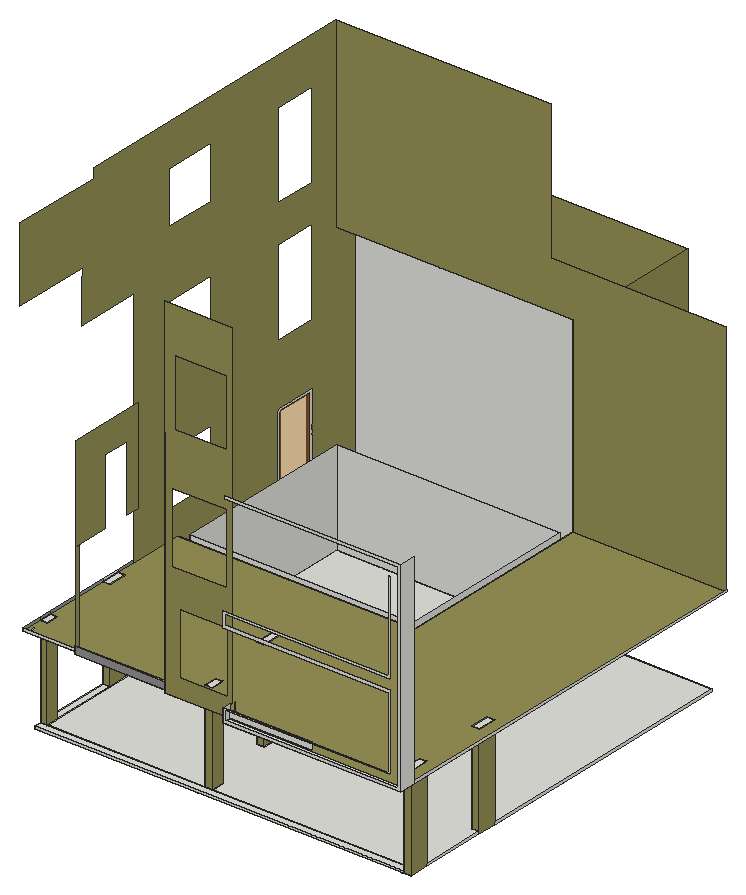
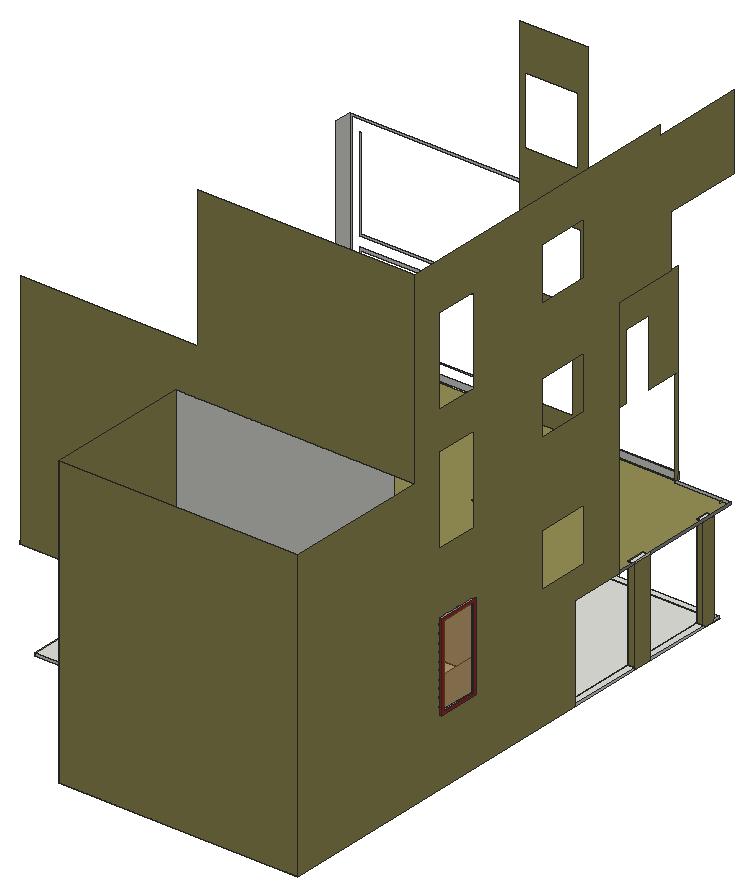
# SketchUp Ruby script. Lengths in inches.
U = 1.inch
M = Sketchup.active_model
def pt(a) = Geom::Point3d.new(a.map { |v| v * U })
def face(e, loops, mat)
  f = e.add_face(loops[0].map { |a| pt(a) })
  loops[1..].each { |l| e.add_face(l.map { |a| pt(a) }).erase! }
  f.material = f.back_material = mat if mat
  f
end
# faces: each face lists its corners as indices into pts; further lists are holes
def faces(e, pts, list, mat = nil) = list.each { |f| face(e, (f[0].is_a?(Array) ? f : [f]).map { |l| l.map { |i| pts[i] } }, mat) }
# xy, xz, yz: faces in a plane at the given z, y or x. An outline is a flat list of corners, or four numbers for a rectangle; further outlines are holes
def ring(l) = l.size == 4 ? [[l[0], l[1]], [l[2], l[1]], [l[2], l[3]], [l[0], l[3]]] : l.each_slice(2).to_a
def flat(e, list, mat, &to3) = list.each { |f| face(e, (f[0].is_a?(Array) ? f : [f]).map { |l| ring(l).map { |u, v| to3.(u, v) } }, mat) }
def xy(e, z, list, mat = nil) = flat(e, list, mat) { |x, y| [x, y, z] }
def xz(e, y, list, mat = nil) = flat(e, list, mat) { |x, z| [x, y, z] }
def yz(e, x, list, mat = nil) = flat(e, list, mat) { |y, z| [x, y, z] }
def lines(e, pts, list) = list.each { |a, b| e.add_line(pt(pts[a]), pt(pts[b])) }
# prism: a flat outline (further loops are holes) pulled along v
def prism(e, loops, v, mat = nil)
  f = face(e, loops, mat); d = Geom::Vector3d.new(v.map { |x| x * U })
  f.pushpull(f.normal.samedirection?(d) ? d.length : -d.length)
end
def box(e, o, s, mat = nil) = prism(e, [[o, [o[0] + s[0], o[1], o[2]], [o[0] + s[0], o[1] + s[1], o[2]], [o[0], o[1] + s[1], o[2]]]], [0, 0, s[2]], mat)
def at(x, y, z, deg = 0) = Geom::Transformation.translation(pt([x, y, z])) * Geom::Transformation.rotation(ORIGIN, Z_AXIS, deg.degrees)
def axes(o, x, y, z) = Geom::Transformation.new([*x, 0, *y, 0, *z, 0, *pt(o).to_a, 1])
def part(name) = M.definitions.add(name)
# library, detail: a bought-in or finely detailed component or shape, given as its bounding box
def library(name, o, s) = part(name).tap { |d| box(d.entities, o, s) }
def detail(e, o, s) = box(e.add_group.entities, o, s)
def put(e, d, t, mat = nil) = e.add_instance(d, t).tap { |i| i.material = mat if mat }
def group(e, t, mat = nil) = e.add_group.tap { |g| g.transformation = t; g.material = mat if mat }.entities
root = M.entities
M.materials.add("[0018_Brown]").color = [165, 42, 42]
M.materials.add("[0057_DarkKhaki]").color = [150, 145, 85]
M.materials.add("[0134_DimGray]").color = [105, 105, 105]
M.materials.add("[Color M05]").color = [145, 145, 145]
M.materials.add("[Translucent Glass Gray]").color = [191, 123, 24]
M.materials["[Translucent Glass Gray]"].alpha = 0.5
xy(root,0,[[12.25,40.75,21.25,40.875],[21.25,40.75,222.625,40.875],[222.625,40.75,482.875,40.875],[11.875,40.875,12.25,65.96],[12.25,40.875,21.25,41.91],
  [21.25,40.875,222.625,49.875],[222.625,40.875,482.875,49.875],[482.875,40.875,491.875,41.91],[12.25,41.91,21.25,49.875],[482.875,41.91,491.875,65.96],
  [12.25,49.875,20.875,65.96],[20.875,49.875,21.25,65.96],[[21.25,49.875,21.25,65.96,20.875,65.96,20.875,268.75,314.375,268.75,314.375,520.875,491.875,520.875,491.875,174.3,482.875,174.3,482.875,150.26,491.875,150.26,491.875,65.96,482.875,65.96,482.875,49.875,231.625,49.875,231.625,65.96,222.625,65.96,222.625,49.875],[208.3125,150.26,217.3125,174.3]],[222.625,49.875,231.625,65.96],[11.875,65.96,20.875,150.26],
  [11.875,150.26,20.875,174.3],[208.3125,150.26,217.3125,174.3],[482.875,150.26,491.875,174.3],[11.875,174.3,20.875,268.75],[[11.875,268.75,314.375,520.875],[20.875,277.75,305.375,511.875]],
  [20.875,277.75,305.375,511.875],[11.875,520.875,38.4375,705.1875],[38.4375,520.875,314.375,705.1875]])
xy(root,3,[[12.25,40.75,482.875,49.875],[[21.25,49.875,222.625,49.875,222.625,65.96,231.625,65.96,231.625,49.875,482.875,49.875,482.875,65.96,491.875,65.96,491.875,150.26,482.875,150.26,482.875,174.3,491.875,174.3,491.875,520.875,314.375,520.875,314.375,268.75,20.875,268.75,20.875,65.96,21.25,65.96],[208.3125,150.26,217.3125,174.3]],[11.875,65.96,20.875,150.26],[11.875,174.3,20.875,268.75]])
xy(root,84.9,[[8.875,428.78,11.875,482.72]],"[0018_Brown]")
xy(root,87.9,[[8.875,431.78,11.875,479.72]],"[0018_Brown]")
xy(root,120,[[284.41,1.0625,510.6875,10.0625],[482.875,41.91,491.875,65.96],[12.25,49.875,20.875,65.96],[222.625,49.875,231.625,65.96],[11.875,150.26,20.875,174.3],
  [208.3125,150.26,217.3125,174.3],[482.875,150.26,491.875,174.3]])
xy(root,120,[[[284.41,10.0625,284.41,12.1875,200.79,12.1875,200.79,18.1875,82.85,18.1875,82.85,22.0625,11.875,22.0625,11.875,150.26,20.875,150.26,20.875,174.3,11.875,174.3,11.875,268.75,314.375,268.75,314.375,520.875,510.6875,520.875,510.6875,10.0625],[482.875,41.91,491.875,65.96],[482.875,150.26,491.875,174.3],[208.3125,150.26,217.3125,174.3],[222.625,49.875,231.625,65.96],[12.25,49.875,20.875,65.96]]],"[0057_DarkKhaki]")
xy(root,120.55,[[82.85,16.375,200.79,18.1875]])
xz(root,1.0625,[[284.41,120,510.6875,120,510.6875,379.43,286.99,379.43,286.99,376.42,507.04,376.42,507.04,123.19,286.64,123.19,286.64,135.48,497.29,135.48,497.29,232.22,286.99,232.22,286.99,244.84,497.49,244.84,497.49,361.64,495.71,361.64,495.71,247.89,284.05,247.89,284.05,228.47,495.71,228.47,495.71,137.03,284.41,137.03]])
xz(root,10.0625,[[286.17,122.27,390.0625,130.6875]])
xz(root,12.1875,[[[200.79,120,284.41,120,284.41,137.03,286.17,137.03,286.17,567.22,200.79,567.22],[209.95,267.29,209.95,357.35,280.45,357.35,280.45,352.16,280.75,352.16,280.75,267.29],[213.98,425.13,213.98,510.5,275.76,510.5,275.76,510.53,279.92,510.53,279.92,425.13],[219.91,142.96,219.91,222.71,281.47,222.71,281.47,219.83,281.16,219.83,281.16,142.96]]],"[0057_DarkKhaki]")
xz(root,16.375,[[82.85,120.55,200.79,129.65]],"[Color M05]")
xz(root,18.1875,[[82.85,120,200.79,120.55],[82.85,120.55,200.79,129.65]])
xz(root,22.0625,[[11.875,120,82.85,123]])
xz(root,40.75,[[12.25,0,482.875,3]])
xz(root,41.91,[[482.875,0,491.875,120]],"[0057_DarkKhaki]")
xz(root,49.875,[[20.875,0,21.25,3],[21.25,0,222.625,3],[222.625,0,231.625,3],[231.625,0,482.875,3]])
xz(root,49.875,[[12.25,0,20.875,3],[12.25,3,20.875,120],[222.625,3,231.625,120]],"[0057_DarkKhaki]")
xz(root,65.96,[[11.875,0,12.25,3],[20.875,0,21.25,3],[222.625,0,231.625,3],[482.875,0,491.875,3]])
xz(root,65.96,[[12.25,0,20.875,3],[12.25,3,20.875,120],[222.625,3,231.625,120],[482.875,3,491.875,120]],"[0057_DarkKhaki]")
xz(root,150.26,[[11.875,0,20.875,3],[208.3125,0,217.3125,3],[482.875,0,491.875,3]])
xz(root,150.26,[[11.875,3,20.875,120],[208.3125,3,217.3125,120],[482.875,3,491.875,120]],"[0057_DarkKhaki]")
xz(root,174.3,[[11.875,0,20.875,3],[208.3125,0,217.3125,3],[482.875,0,491.875,3]])
xz(root,174.3,[[11.875,3,20.875,120],[208.3125,3,217.3125,120],[482.875,3,491.875,120]],"[0057_DarkKhaki]")
xz(root,268.75,[[11.875,0,20.875,3],[20.875,0,314.375,3]])
xz(root,268.75,[[11.875,3,314.375,120]],"[0057_DarkKhaki]")
xz(root,277.75,[[20.875,0,305.375,120]])
xz(root,428.78,[[8.875,84.9,11.875,194.21]],"[0018_Brown]")
xz(root,431.78,[[8.875,87.9,11.875,191.21]],"[0018_Brown]")
xz(root,479.72,[[8.875,87.9,11.875,191.21]],"[0018_Brown]")
xz(root,482.72,[[8.875,84.9,11.875,194.21]],"[0018_Brown]")
xz(root,511.875,[[20.875,0,305.375,120]])
xz(root,520.875,[[38.4375,0,314.375,363],[314.375,0,491.875,3]])
xz(root,520.875,[[314.375,120,314.375,363,11.875,363,11.875,599.125,286.17,599.125,286.17,423,509.75,423,509.75,123,510.6875,123,510.6875,120]],"[0057_DarkKhaki]")
xz(root,705.1875,[[11.875,0,314.375,363]],"[0057_DarkKhaki]")
yz(root,8.875,[[[428.78,84.9,482.72,194.21],[431.78,87.9,479.72,191.21]]],"[0018_Brown]")
yz(root,11.875,[[65.96,0,150.26,3],[174.3,0,268.75,3],[[428.78,84.9,482.72,194.21],[431.78,87.9,479.72,191.21]],[150.26,120,174.3,123]])
yz(root,11.875,[[[268.75,0,268.75,120,199.5,120,199.5,426.78,116.75,426.78,116.75,483,117.1875,483,117.1875,493.0625,18.1875,493.0625,18.1875,587.3125,135.0625,587.3125,135.0625,599.125,520.875,599.125,520.875,363,705.1875,363,705.1875,0],[428.78,84.9,482.72,194.21],[428.78,273.08,482.72,382.4],[428.78,429.83,482.72,539.15],[254.47,155.78,321.35,222.65],[254.47,327.4,321.35,394.28],[254.47,479.03,321.35,545.9]],[150.26,0,174.3,120]],"[0057_DarkKhaki]")
yz(root,11.875,[[22.0625,120,150.26,123],[150.26,120,174.3,123],[174.3,120,199.5,123]],"[Color M05]")
yz(root,11.875,[[431.78,87.9,479.72,191.21]],"[Translucent Glass Gray]")
yz(root,12.25,[[40.75,0,49.875,3]])
yz(root,12.25,[[49.875,0,65.96,120]],"[0057_DarkKhaki]")
yz(root,20.875,[[65.96,0,150.26,3],[150.26,0,174.3,3],[174.3,0,268.75,3],[277.75,0,511.875,120],[27.125,121.9375,27.5625,121.99,27.97,122.16,28.32,122.43,28.59,122.78,28.68,123,25.57,123,25.66,122.78,25.93,122.43,26.28,122.16,26.6875,121.99]])
yz(root,20.875,[[49.875,0,65.96,120],[150.26,3,174.3,120]],"[0057_DarkKhaki]")
yz(root,21.25,[[49.875,0,65.96,3]])
yz(root,82.85,[[18.1875,120,18.1875,363.37,116.75,363.37,116.75,243,99.65,243,99.65,327,63.65,327,63.65,243,22.0625,243,22.0625,243.17,19.6875,243.17,19.6875,242.08,22.0625,242.08,22.0625,120]],"[0057_DarkKhaki]")
yz(root,82.85,[[16.375,120.55,18.1875,129.65]],"[Color M05]")
yz(root,200.79,[[16.375,120.55,18.1875,129.65]])
yz(root,200.79,[[12.1875,120,12.1875,417.72,18.1875,417.72,18.1875,417.65,15.1875,417.65,15.1875,408.55,18.1875,408.55,18.1875,405.65,15.1875,405.65,15.1875,396.55,18.1875,396.55,18.1875,393.65,15.1875,393.65,15.1875,384.55,18.1875,384.55,18.1875,381.65,15.1875,381.65,15.1875,372.55,18.1875,372.55,18.1875,369.65,15.1875,369.65,15.1875,360.55,18.1875,360.55,18.1875,357.65,15.1875,357.65,15.1875,348.55,18.1875,348.55,18.1875,345.65,15.1875,345.65,15.1875,336.55,18.1875,336.55,18.1875,333.65,15.1875,333.65,15.1875,324.55,18.1875,324.55,18.1875,321.65,15.1875,321.65,15.1875,312.55,18.1875,312.55,18.1875,309.65,15.1875,309.65,15.1875,300.55,18.1875,300.55,18.1875,297.65,15.1875,297.65,15.1875,288.55,18.1875,288.55,18.1875,285.65,15.1875,285.65,15.1875,276.55,18.1875,276.55,18.1875,273.65,15.1875,273.65,15.1875,264.55,18.1875,264.55,18.1875,261.65,15.1875,261.65,15.1875,252.55,18.1875,252.55,18.1875,249.65,15.1875,249.65,15.1875,240.55,18.1875,240.55,18.1875,237.65,15.1875,237.65,15.1875,228.55,18.1875,228.55,18.1875,225.65,15.1875,225.65,15.1875,216.55,18.1875,216.55,18.1875,213.65,15.1875,213.65,15.1875,204.55,18.1875,204.55,18.1875,201.65,15.1875,201.65,15.1875,192.55,18.1875,192.55,18.1875,189.65,15.1875,189.65,15.1875,180.55,18.1875,180.55,18.1875,177.65,16.375,177.65,16.375,168.55,18.1875,168.55,18.1875,165.65,16.375,165.65,16.375,156.55,18.1875,156.55,18.1875,153.65,16.375,153.65,16.375,144.55,18.1875,144.55,18.1875,141.65,16.375,141.65,16.375,132.55,18.1875,132.55,18.1875,129.65,16.375,129.65,16.375,120.55,18.1875,120.55,18.1875,120]],"[0134_DimGray]")
yz(root,208.3125,[[150.26,0,174.3,3]])
yz(root,208.3125,[[150.26,3,174.3,120]],"[0057_DarkKhaki]")
yz(root,217.3125,[[150.26,0,174.3,3]])
yz(root,217.3125,[[150.26,3,174.3,120]],"[0057_DarkKhaki]")
yz(root,222.625,[[49.875,0,65.96,3]])
yz(root,222.625,[[49.875,3,65.96,120]],"[0057_DarkKhaki]")
yz(root,231.625,[[49.875,0,65.96,3]])
yz(root,231.625,[[49.875,3,65.96,120]],"[0057_DarkKhaki]")
yz(root,284.41,[[1.0625,120,12.1875,135.98]])
yz(root,305.375,[[277.75,0,511.875,120]])
yz(root,314.375,[[268.75,0,520.875,3]])
yz(root,314.375,[[520.875,0,705.1875,363],[268.75,3,520.875,120]],"[0057_DarkKhaki]")
yz(root,482.875,[[40.75,0,41.91,3],[49.875,0,65.96,3],[150.26,0,174.3,3]])
yz(root,482.875,[[41.91,0,49.875,3],[41.91,3,65.96,120],[150.26,3,174.3,120]],"[0057_DarkKhaki]")
yz(root,491.875,[[65.96,0,150.26,3],[174.3,0,520.875,3]])
yz(root,491.875,[[41.91,0,65.96,120],[150.26,0,174.3,120]],"[0057_DarkKhaki]")
yz(root,510.6875,[[1.0625,120,22.0625,379.43],[22.0625,120,520.875,123]])
p = [[12.25,65.96,120],[12.25,65.96,123],[12.25,49.875,120],[12.25,49.875,123],[216.79,22.0625,123],[216.79,22.0625,120],
  [216.73,22.0625,123],[284.41,22.0625,123],[284.41,22.0625,120],[284.41,18.1875,135.98],[284.41,18.1875,120],[286.17,18.1875,137.03],
  [286.17,18.1875,120],[11.875,199.5,120],[11.875,199.5,118.82]]
lines(root,p,[[0,1],[2,3],[4,5],[6,5],[7,8],[9,10],[11,12],[13,14]])
